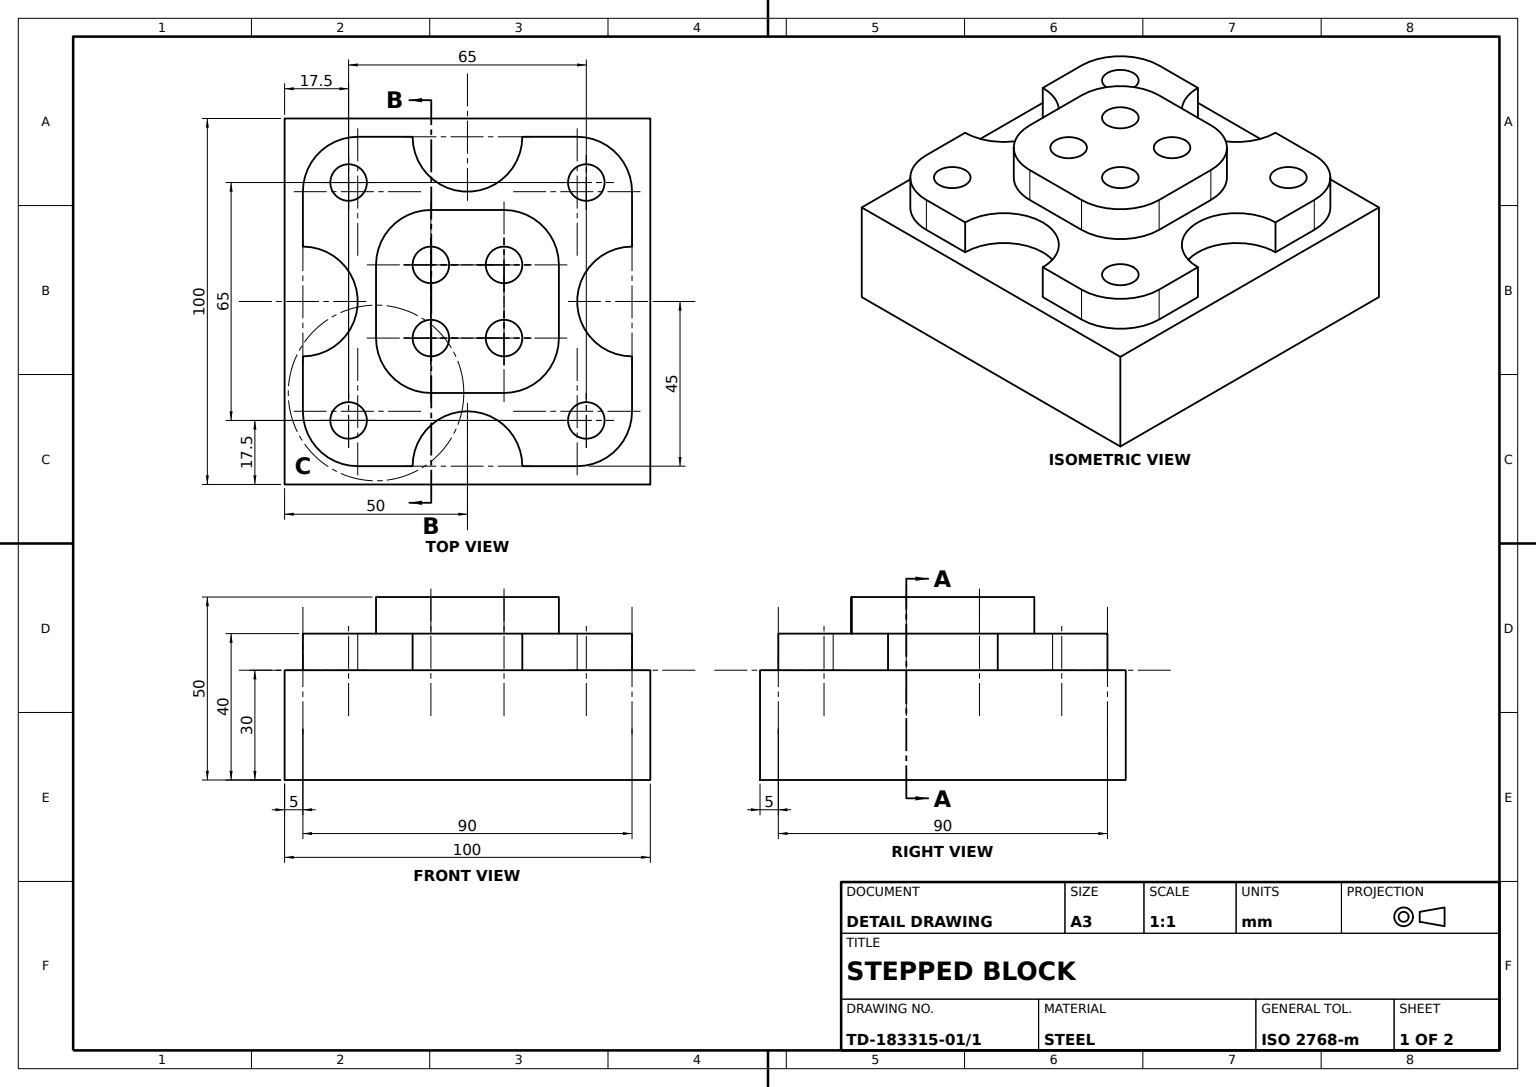
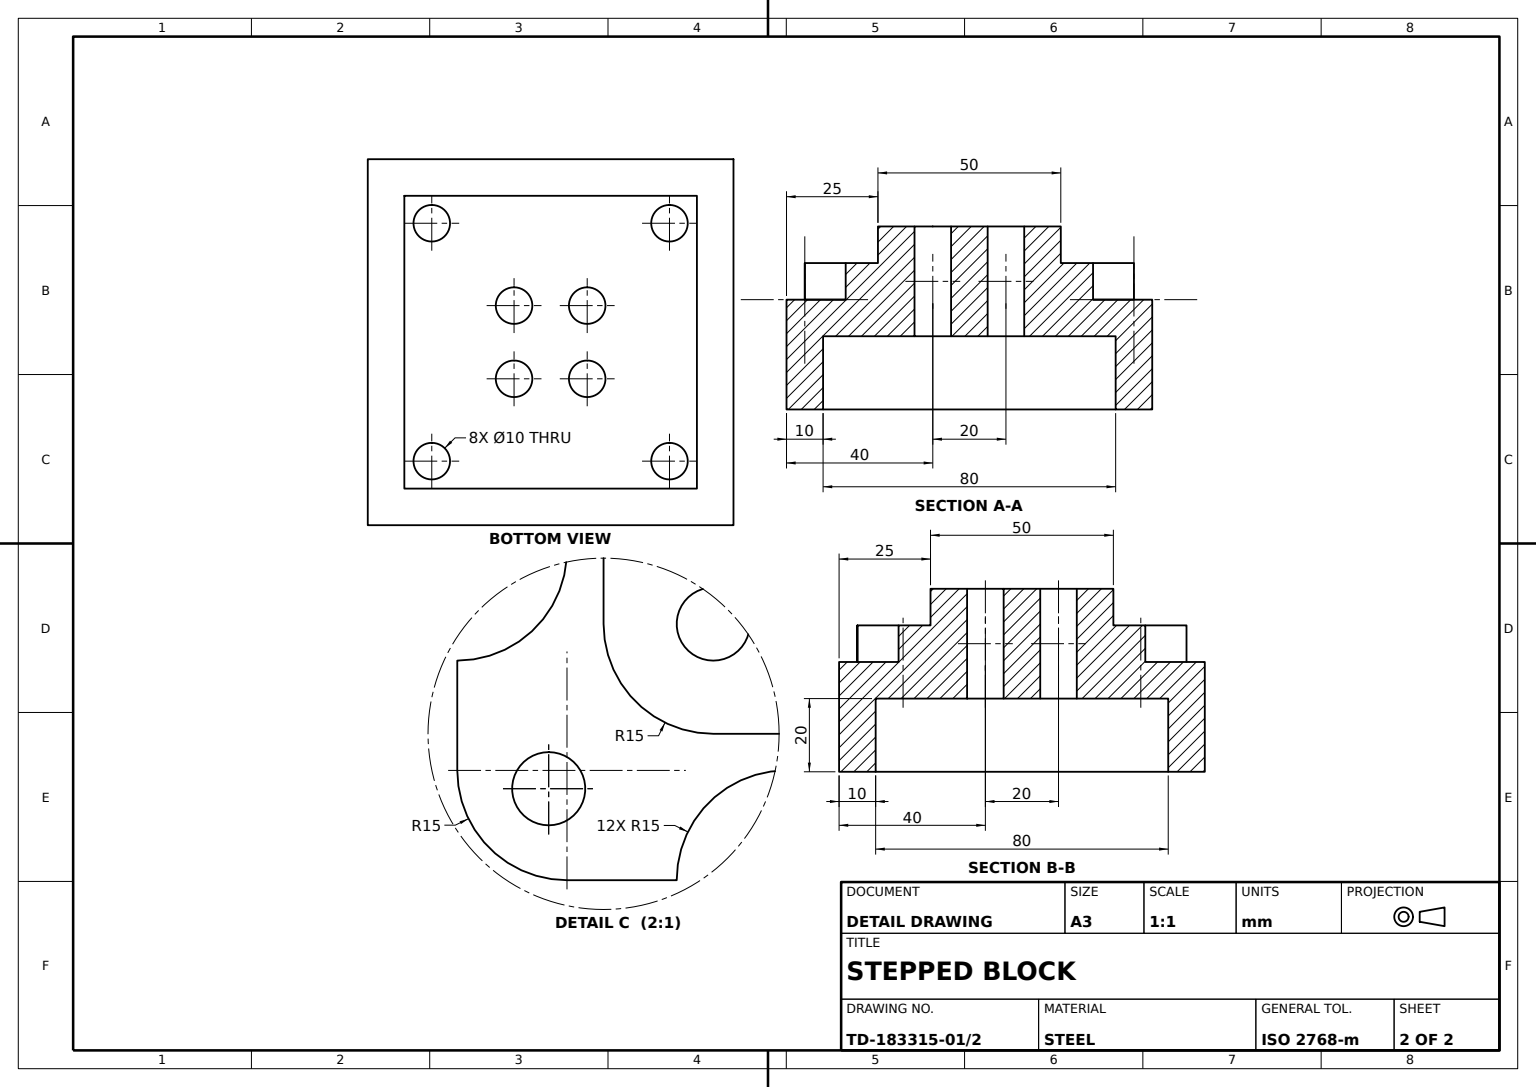
solid
v1 (40,0,40)
v2 (40,0,-40)
e1 v1 v2 LINE
v3 (40,20,40)
e2 v3 v1 LINE
v4 (40,20,-40)
e3 v3 v4 LINE
e4 v4 v2 LINE
face PLANE(AX(P(40,30,50),D(-1,0,0),D(0,0,1))) [-e1 -e2 e3 e4]
v5 (45,40,30)
v6 (45,30,30)
e5 v5 v6 LINE
v7 (45,30,15)
e6 v6 v7 LINE
v8 (45,40,15)
e7 v8 v7 LINE
e8 v5 v8 LINE
face PLANE(AX(P(45,40,30),D(-1,0,0),D(0,0,1))) rev [e5 e6 -e7 -e8]
v9 (-32.5,20,-37.5)
v10 (-32.5,20,-27.5)
e9 v9 v10 CIRCLE(AX(P(-32.5,20,-32.5),D(0,-1,0),D(0,0,-1)),5)
v11 (-32.5,40,-27.5)
e10 v11 v10 LINE
v12 (-32.5,40,-37.5)
e11 v11 v12 CIRCLE(AX(P(-32.5,40,-32.5),D(0,1,0),D(0,0,1)),5)
e12 v12 v9 LINE
face CYL(AX(P(-32.5,40,-32.5),D(0,-1,0),D(0,0,-1)),5) rev [e9 -e10 e11 e12]
v13 (45,40,-15)
v14 (45,30,-15)
e13 v13 v14 LINE
v15 (45,30,-30)
e14 v14 v15 LINE
v16 (45,40,-30)
e15 v16 v15 LINE
e16 v13 v16 LINE
face PLANE(AX(P(45,40,-15),D(-1,0,0),D(0,0,1))) rev [e13 e14 -e15 -e16]
v17 (10,50,-15)
v18 (10,50,-5)
e17 v17 v18 CIRCLE(AX(P(10,50,-10),D(0,1,0),D(0,0,1)),5)
v19 (10,20,-5)
e18 v18 v19 LINE
v20 (10,20,-15)
e19 v19 v20 CIRCLE(AX(P(10,20,-10),D(0,-1,0),D(0,0,-1)),5)
e20 v17 v20 LINE
face CYL(AX(P(10,50,-10),D(0,-1,0),D(0,0,-1)),5) rev [e17 e18 e19 -e20]
v21 (32.5,40,37.5)
v22 (32.5,20,37.5)
e21 v21 v22 LINE
v23 (32.5,40,27.5)
e22 v21 v23 CIRCLE(AX(P(32.5,40,32.5),D(0,1,0),D(0,0,1)),5)
v24 (32.5,20,27.5)
e23 v23 v24 LINE
e24 v24 v22 CIRCLE(AX(P(32.5,20,32.5),D(0,-1,0),D(0,0,-1)),5)
face CYL(AX(P(32.5,40,32.5),D(0,-1,0),D(0,0,-1)),5) rev [-e21 e22 e23 e24]
v25 (-45,40,-30)
v26 (-45,30,-30)
e25 v25 v26 LINE
v27 (-45,30,-15)
e26 v26 v27 LINE
v28 (-45,40,-15)
e27 v28 v27 LINE
e28 v25 v28 LINE
face PLANE(AX(P(-45,40,-15),D(1,0,0),D(0,0,-1))) rev [e25 e26 -e27 -e28]
e29 v23 v21 CIRCLE(AX(P(32.5,40,32.5),D(0,1,0),D(0,0,1)),5)
e30 v22 v24 CIRCLE(AX(P(32.5,20,32.5),D(0,-1,0),D(0,0,-1)),5)
face CYL(AX(P(32.5,40,32.5),D(0,-1,0),D(0,0,-1)),5) rev [-e23 e29 e21 e30]
e31 v12 v11 CIRCLE(AX(P(-32.5,40,-32.5),D(0,1,0),D(0,0,1)),5)
e32 v10 v9 CIRCLE(AX(P(-32.5,20,-32.5),D(0,-1,0),D(0,0,-1)),5)
face CYL(AX(P(-32.5,40,-32.5),D(0,-1,0),D(0,0,-1)),5) rev [e31 e10 e32 -e12]
v29 (-32.5,40,37.5)
v30 (-32.5,20,37.5)
e33 v29 v30 LINE
v31 (-32.5,40,27.5)
e34 v29 v31 CIRCLE(AX(P(-32.5,40,32.5),D(0,1,0),D(0,0,1)),5)
v32 (-32.5,20,27.5)
e35 v31 v32 LINE
e36 v32 v30 CIRCLE(AX(P(-32.5,20,32.5),D(0,-1,0),D(0,0,-1)),5)
face CYL(AX(P(-32.5,40,32.5),D(0,-1,0),D(0,0,-1)),5) rev [-e33 e34 e35 e36]
v33 (30,40,45)
v34 (30,30,45)
e37 v33 v34 LINE
v35 (15,40,45)
e38 v35 v33 LINE
v36 (15,30,45)
e39 v35 v36 LINE
e40 v36 v34 LINE
face PLANE(AX(P(15,40,45),D(0,0,-1),D(-1,0,0))) rev [-e37 -e38 e39 e40]
v37 (-15,40,45)
v38 (-15,30,45)
e41 v37 v38 LINE
v39 (-30,40,45)
e42 v39 v37 LINE
v40 (-30,30,45)
e43 v39 v40 LINE
e44 v40 v38 LINE
face PLANE(AX(P(-30,40,45),D(0,0,-1),D(-1,0,0))) rev [-e41 -e42 e43 e44]
v41 (-45,40,30)
v42 (-45,30,30)
e45 v41 v42 LINE
e46 v42 v40 CIRCLE(AX(P(-30,30,30),D(0,1,0),D(0,0,-1)),15)
e47 v41 v39 CIRCLE(AX(P(-30,40,30),D(0,1,0),D(0,0,-1)),15)
face CYL(AX(P(-30,40,30),D(0,-1,0),D(0,0,-1)),15) [e45 e46 -e43 -e47]
v43 (-10,50,-25)
v44 (-25,50,-10)
e48 v43 v44 CIRCLE(AX(P(-10,50,-10),D(0,1,0),D(0,0,1)),15)
v45 (-10,40,-25)
e49 v43 v45 LINE
v46 (-25,40,-10)
e50 v45 v46 CIRCLE(AX(P(-10,40,-10),D(0,1,0),D(0,0,1)),15)
e51 v44 v46 LINE
face CYL(AX(P(-10,50,-10),D(0,-1,0),D(0,0,-1)),15) [-e48 e49 e50 -e51]
e52 v8 v13 CIRCLE(AX(P(45,40,0),D(0,-1,0),D(0,0,1)),15)
e53 v7 v14 CIRCLE(AX(P(45,30,0),D(0,-1,0),D(0,0,1)),15)
face CYL(AX(P(45,40,0),D(0,-1,0),D(0,0,-1)),15) rev [-e13 -e52 e7 e53]
v47 (0,40,30)
v48 (0,30,30)
e54 v47 v48 LINE
e55 v37 v47 CIRCLE(AX(P(0,40,45),D(0,-1,0),D(0,0,1)),15)
e56 v38 v48 CIRCLE(AX(P(0,30,45),D(0,-1,0),D(0,0,1)),15)
face CYL(AX(P(0,40,45),D(0,-1,0),D(0,0,-1)),15) rev [-e54 -e55 e41 e56]
v49 (-25,40,10)
e57 v46 v49 LINE
v50 (-25,50,10)
e58 v50 v49 LINE
e59 v44 v50 LINE
face PLANE(AX(P(-25,50,-10),D(1,0,0),D(0,0,-1))) rev [e51 e57 -e58 -e59]
v51 (-10,20,15)
v52 (-10,20,5)
e60 v51 v52 CIRCLE(AX(P(-10,20,10),D(0,-1,0),D(0,0,-1)),5)
v53 (-10,50,5)
e61 v53 v52 LINE
v54 (-10,50,15)
e62 v53 v54 CIRCLE(AX(P(-10,50,10),D(0,1,0),D(0,0,1)),5)
e63 v54 v51 LINE
face CYL(AX(P(-10,50,10),D(0,-1,0),D(0,0,-1)),5) rev [e60 -e61 e62 e63]
v55 (15,30,-45)
v56 (-15,30,-45)
e64 v55 v56 CIRCLE(AX(P(0,30,-45),D(0,-1,0),D(0,0,1)),15)
v57 (-15,40,-45)
e65 v57 v56 LINE
v58 (15,40,-45)
e66 v58 v57 CIRCLE(AX(P(0,40,-45),D(0,-1,0),D(0,0,1)),15)
e67 v58 v55 LINE
face CYL(AX(P(0,40,-45),D(0,-1,0),D(0,0,-1)),15) rev [e64 -e65 -e66 e67]
e68 v20 v19 CIRCLE(AX(P(10,20,-10),D(0,-1,0),D(0,0,-1)),5)
e69 v18 v17 CIRCLE(AX(P(10,50,-10),D(0,1,0),D(0,0,1)),5)
face CYL(AX(P(10,50,-10),D(0,-1,0),D(0,0,-1)),5) rev [e68 -e18 e69 e20]
v59 (30,40,-45)
e70 v59 v58 LINE
v60 (30,30,-45)
e71 v59 v60 LINE
e72 v60 v55 LINE
face PLANE(AX(P(15,40,-45),D(0,0,1),D(1,0,0))) rev [-e70 e71 e72 -e67]
v61 (-40,20,40)
v62 (-40,0,40)
e73 v61 v62 LINE
e74 v61 v3 LINE
e75 v62 v1 LINE
face PLANE(AX(P(-50,30,40),D(0,0,-1),D(-1,0,0))) [-e73 e74 e2 -e75]
v63 (-50,30,-50)
v64 (-50,30,50)
e76 v63 v64 LINE
v65 (-50,0,-50)
e77 v63 v65 LINE
v66 (-50,0,50)
e78 v65 v66 LINE
e79 v64 v66 LINE
face PLANE(AX(P(-50,30,50),D(1,0,0),D(0,0,-1))) rev [-e76 e77 e78 -e79]
e80 v48 v36 CIRCLE(AX(P(0,30,45),D(0,-1,0),D(0,0,1)),15)
e81 v47 v35 CIRCLE(AX(P(0,40,45),D(0,-1,0),D(0,0,1)),15)
face CYL(AX(P(0,40,45),D(0,-1,0),D(0,0,-1)),15) rev [e54 e80 -e39 -e81]
e82 v31 v29 CIRCLE(AX(P(-32.5,40,32.5),D(0,1,0),D(0,0,1)),5)
v67 (32.5,40,-37.5)
v68 (32.5,40,-27.5)
e83 v67 v68 CIRCLE(AX(P(32.5,40,-32.5),D(0,1,0),D(0,0,1)),5)
e84 v68 v67 CIRCLE(AX(P(32.5,40,-32.5),D(0,1,0),D(0,0,1)),5)
v69 (10,40,-25)
e85 v69 v45 LINE
v70 (25,40,-10)
e86 v70 v69 CIRCLE(AX(P(10,40,-10),D(0,1,0),D(0,0,1)),15)
v71 (25,40,10)
e87 v71 v70 LINE
v72 (10,40,25)
e88 v72 v71 CIRCLE(AX(P(10,40,10),D(0,1,0),D(0,0,1)),15)
v73 (-10,40,25)
e89 v73 v72 LINE
e90 v49 v73 CIRCLE(AX(P(-10,40,10),D(0,1,0),D(0,0,1)),15)
e91 v33 v5 CIRCLE(AX(P(30,40,30),D(0,1,0),D(0,0,1)),15)
e92 v16 v59 CIRCLE(AX(P(30,40,-30),D(0,1,0),D(0,0,-1)),15)
v74 (-30,40,-45)
e93 v57 v74 LINE
e94 v74 v25 CIRCLE(AX(P(-30,40,-30),D(0,1,0),D(0,0,-1)),15)
v75 (-45,40,15)
e95 v28 v75 CIRCLE(AX(P(-45,40,0),D(0,-1,0),D(0,0,1)),15)
e96 v75 v41 LINE
face PLANE(AX(P(-30,40,30),D(0,-1,0),D(0,0,-1))) rev [-e31 -e11] [-e82 -e34] [-e83 -e84] [-e50 -e85 -e86 -e87 -e88 -e89 -e90 -e57] [-e22 -e29] [e81 e38 e91 e8 e52 e16 e92 e70 e66 e93 e94 e28 e95 e96 e47 e42 e55]
v76 (32.5,20,-27.5)
e97 v68 v76 LINE
v77 (32.5,20,-37.5)
e98 v67 v77 LINE
e99 v77 v76 CIRCLE(AX(P(32.5,20,-32.5),D(0,-1,0),D(0,0,-1)),5)
face CYL(AX(P(32.5,40,-32.5),D(0,-1,0),D(0,0,-1)),5) rev [-e97 e84 e98 e99]
v78 (-30,30,-45)
e100 v56 v78 LINE
e101 v74 v78 LINE
face PLANE(AX(P(-30,40,-45),D(0,0,1),D(1,0,0))) rev [-e93 e65 e100 -e101]
v79 (50,30,-50)
v80 (50,0,-50)
e102 v79 v80 LINE
e103 v80 v65 LINE
e104 v79 v63 LINE
face PLANE(AX(P(-50,30,-50),D(0,0,1),D(1,0,0))) rev [e102 e103 -e77 -e104]
e105 v15 v60 CIRCLE(AX(P(30,30,-30),D(0,1,0),D(0,0,-1)),15)
face CYL(AX(P(30,40,-30),D(0,-1,0),D(0,0,-1)),15) [-e92 e15 e105 -e71]
v81 (50,30,50)
e106 v64 v81 LINE
v82 (50,0,50)
e107 v66 v82 LINE
e108 v81 v82 LINE
face PLANE(AX(P(-50,30,50),D(0,0,-1),D(-1,0,0))) rev [-e106 e79 e107 -e108]
e109 v76 v77 CIRCLE(AX(P(32.5,20,-32.5),D(0,-1,0),D(0,0,-1)),5)
face CYL(AX(P(32.5,40,-32.5),D(0,-1,0),D(0,0,-1)),5) rev [e97 e109 -e98 e83]
v83 (-40,0,-40)
e110 v83 v62 LINE
e111 v2 v83 LINE
e112 v82 v80 LINE
face PLANE(AX(P(0,0,0),D(0,-1,0),D(0,0,-1))) [e110 e75 e1 e111] [-e107 -e78 -e103 -e112]
v84 (-45,30,15)
e113 v75 v84 LINE
e114 v84 v42 LINE
face PLANE(AX(P(-45,40,30),D(1,0,0),D(0,0,-1))) rev [-e45 -e96 e113 e114]
v85 (10,50,5)
v86 (10,20,5)
e115 v85 v86 LINE
v87 (10,20,15)
e116 v86 v87 CIRCLE(AX(P(10,20,10),D(0,-1,0),D(0,0,-1)),5)
v88 (10,50,15)
e117 v88 v87 LINE
e118 v88 v85 CIRCLE(AX(P(10,50,10),D(0,1,0),D(0,0,1)),5)
face CYL(AX(P(10,50,10),D(0,-1,0),D(0,0,-1)),5) rev [e115 e116 -e117 e118]
e119 v85 v88 CIRCLE(AX(P(10,50,10),D(0,1,0),D(0,0,1)),5)
e120 v87 v86 CIRCLE(AX(P(10,20,10),D(0,-1,0),D(0,0,-1)),5)
face CYL(AX(P(10,50,10),D(0,-1,0),D(0,0,-1)),5) rev [e119 e117 e120 -e115]
e121 v81 v79 LINE
e122 v34 v6 CIRCLE(AX(P(30,30,30),D(0,1,0),D(0,0,1)),15)
e123 v27 v84 CIRCLE(AX(P(-45,30,0),D(0,-1,0),D(0,0,1)),15)
e124 v78 v26 CIRCLE(AX(P(-30,30,-30),D(0,1,0),D(0,0,-1)),15)
face PLANE(AX(P(0,30,0),D(0,-1,0),D(0,0,-1))) rev [e76 e106 e121 e104] [-e64 -e72 -e105 -e14 -e53 -e6 -e122 -e40 -e80 -e56 -e44 -e46 -e114 -e123 -e26 -e124 -e100]
v89 (25,50,-10)
v90 (10,50,-25)
e125 v89 v90 CIRCLE(AX(P(10,50,-10),D(0,1,0),D(0,0,1)),15)
e126 v89 v70 LINE
e127 v90 v69 LINE
face CYL(AX(P(10,50,-10),D(0,-1,0),D(0,0,-1)),15) [-e125 e126 e86 -e127]
face CYL(AX(P(30,40,30),D(0,-1,0),D(0,0,-1)),15) [e37 e122 -e5 -e91]
v91 (25,50,10)
e128 v91 v89 LINE
e129 v91 v71 LINE
face PLANE(AX(P(25,50,-10),D(-1,0,0),D(0,0,1))) rev [-e126 -e128 e129 e87]
e130 v52 v51 CIRCLE(AX(P(-10,20,10),D(0,-1,0),D(0,0,-1)),5)
e131 v54 v53 CIRCLE(AX(P(-10,50,10),D(0,1,0),D(0,0,1)),5)
face CYL(AX(P(-10,50,10),D(0,-1,0),D(0,0,-1)),5) rev [e130 -e63 e131 e61]
v92 (-10,50,-15)
v93 (-10,50,-5)
e132 v92 v93 CIRCLE(AX(P(-10,50,-10),D(0,1,0),D(0,0,1)),5)
e133 v93 v92 CIRCLE(AX(P(-10,50,-10),D(0,1,0),D(0,0,1)),5)
v94 (10,50,25)
e134 v94 v91 CIRCLE(AX(P(10,50,10),D(0,1,0),D(0,0,1)),15)
e135 v90 v43 LINE
v95 (-10,50,25)
e136 v50 v95 CIRCLE(AX(P(-10,50,10),D(0,1,0),D(0,0,1)),15)
e137 v95 v94 LINE
face PLANE(AX(P(-10,50,-10),D(0,1,0),D(0,0,1))) [-e118 -e119] [-e17 -e69] [-e132 -e133] [-e62 -e131] [e134 e128 e125 e135 e48 e59 e136 e137]
face PLANE(AX(P(-10,50,-25),D(0,0,1),D(1,0,0))) rev [-e49 -e135 e127 e85]
face CYL(AX(P(-45,40,0),D(0,-1,0),D(0,0,-1)),15) rev [-e95 e27 e123 -e113]
e138 v94 v72 LINE
e139 v95 v73 LINE
face PLANE(AX(P(-10,50,25),D(0,0,-1),D(-1,0,0))) rev [-e138 -e137 e139 e89]
e140 v30 v32 CIRCLE(AX(P(-32.5,20,32.5),D(0,-1,0),D(0,0,-1)),5)
face CYL(AX(P(-32.5,40,32.5),D(0,-1,0),D(0,0,-1)),5) rev [e82 e33 e140 -e35]
v96 (-10,20,-15)
v97 (-10,20,-5)
e141 v96 v97 CIRCLE(AX(P(-10,20,-10),D(0,-1,0),D(0,0,-1)),5)
e142 v97 v96 CIRCLE(AX(P(-10,20,-10),D(0,-1,0),D(0,0,-1)),5)
v98 (-40,20,-40)
e143 v98 v61 LINE
e144 v4 v98 LINE
face PLANE(AX(P(0,20,0),D(0,-1,0),D(0,0,-1))) [-e99 -e109] [-e130 -e60] [-e141 -e142] [-e32 -e9] [-e30 -e24] [-e140 -e36] [-e68 -e19] [-e74 -e143 -e144 -e3] [-e120 -e116]
face PLANE(AX(P(50,30,50),D(-1,0,0),D(0,0,1))) rev [-e102 -e121 e108 e112]
e145 v98 v83 LINE
face PLANE(AX(P(-50,30,-40),D(0,0,1),D(1,0,0))) [e144 e145 -e111 -e4]
face PLANE(AX(P(-40,30,50),D(1,0,0),D(0,0,-1))) [e73 -e110 -e145 e143]
face CYL(AX(P(-10,50,10),D(0,-1,0),D(0,0,-1)),15) [-e139 -e136 e58 e90]
face CYL(AX(P(10,50,10),D(0,-1,0),D(0,0,-1)),15) [-e129 -e134 e138 e88]
face CYL(AX(P(-30,40,-30),D(0,-1,0),D(0,0,-1)),15) [-e25 -e94 e101 e124]
e146 v93 v97 LINE
e147 v92 v96 LINE
face CYL(AX(P(-10,50,-10),D(0,-1,0),D(0,0,-1)),5) rev [e141 -e146 e133 e147]
face CYL(AX(P(-10,50,-10),D(0,-1,0),D(0,0,-1)),5) rev [-e147 e132 e146 e142]
